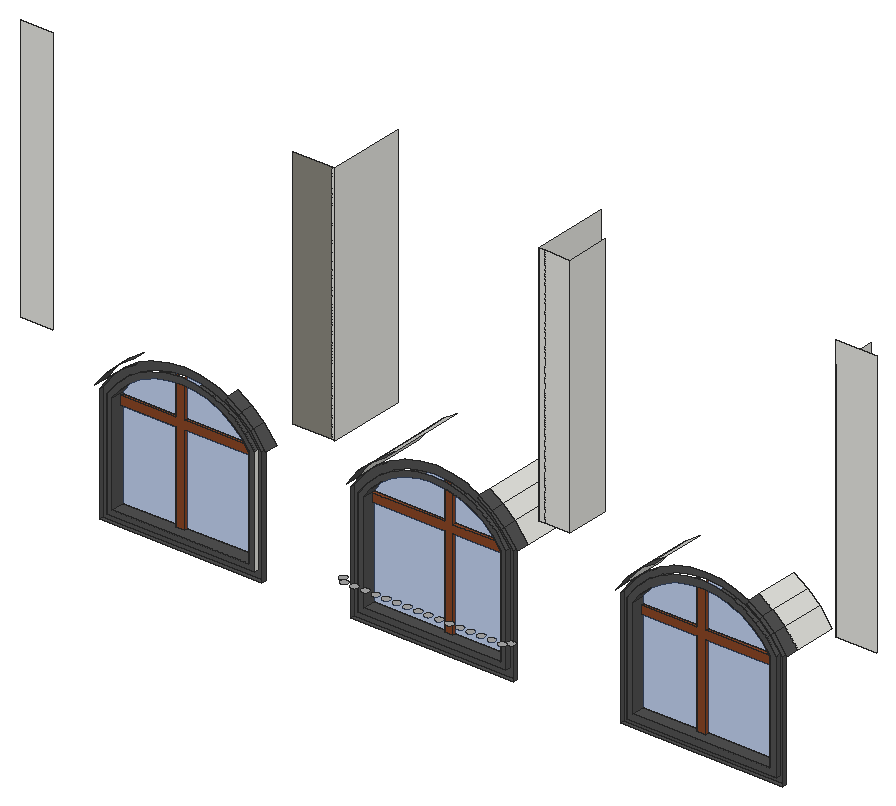
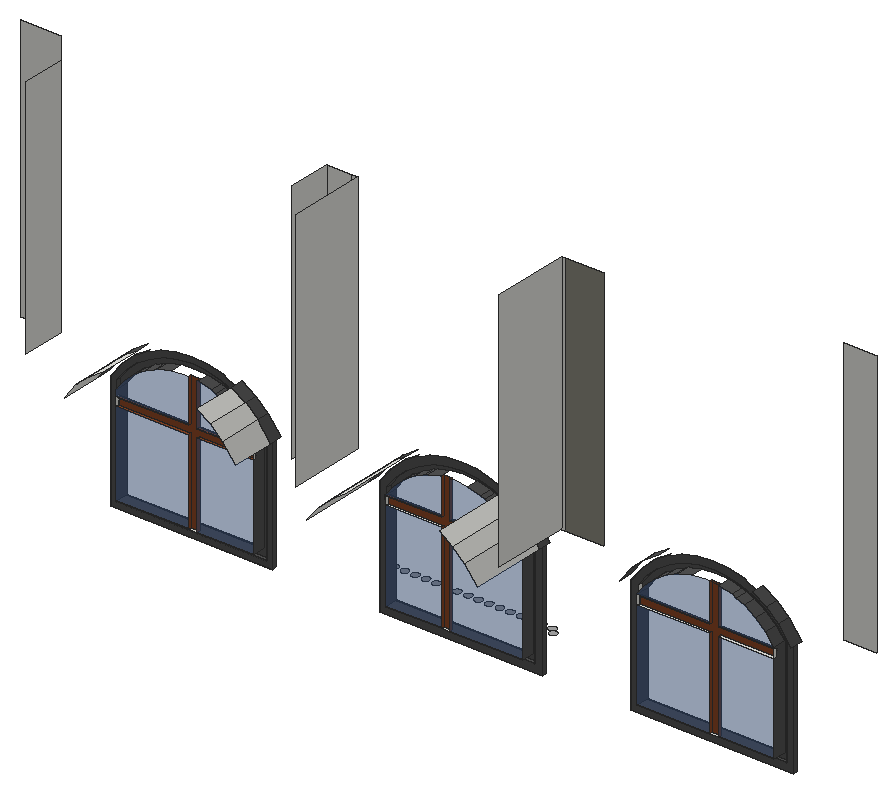
# SketchUp Ruby script. Lengths in inches.
U = 1.inch
M = Sketchup.active_model
def pt(a) = Geom::Point3d.new(a.map { |v| v * U })
def face(e, loops, mat)
  f = e.add_face(loops[0].map { |a| pt(a) })
  loops[1..].each { |l| e.add_face(l.map { |a| pt(a) }).erase! }
  f.material = f.back_material = mat if mat
  f
end
# faces: each face lists its corners as indices into pts; further lists are holes
def faces(e, pts, list, mat = nil) = list.each { |f| face(e, (f[0].is_a?(Array) ? f : [f]).map { |l| l.map { |i| pts[i] } }, mat) }
# xy, xz, yz: faces in a plane at the given z, y or x. An outline is a flat list of corners, or four numbers for a rectangle; further outlines are holes
def ring(l) = l.size == 4 ? [[l[0], l[1]], [l[2], l[1]], [l[2], l[3]], [l[0], l[3]]] : l.each_slice(2).to_a
def flat(e, list, mat, &to3) = list.each { |f| face(e, (f[0].is_a?(Array) ? f : [f]).map { |l| ring(l).map { |u, v| to3.(u, v) } }, mat) }
def xy(e, z, list, mat = nil) = flat(e, list, mat) { |x, y| [x, y, z] }
def xz(e, y, list, mat = nil) = flat(e, list, mat) { |x, z| [x, y, z] }
def yz(e, x, list, mat = nil) = flat(e, list, mat) { |y, z| [x, y, z] }
def lines(e, pts, list) = list.each { |a, b| e.add_line(pt(pts[a]), pt(pts[b])) }
# prism: a flat outline (further loops are holes) pulled along v
def prism(e, loops, v, mat = nil)
  f = face(e, loops, mat); d = Geom::Vector3d.new(v.map { |x| x * U })
  f.pushpull(f.normal.samedirection?(d) ? d.length : -d.length)
end
def box(e, o, s, mat = nil) = prism(e, [[o, [o[0] + s[0], o[1], o[2]], [o[0] + s[0], o[1] + s[1], o[2]], [o[0], o[1] + s[1], o[2]]]], [0, 0, s[2]], mat)
def at(x, y, z, deg = 0) = Geom::Transformation.translation(pt([x, y, z])) * Geom::Transformation.rotation(ORIGIN, Z_AXIS, deg.degrees)
def axes(o, x, y, z) = Geom::Transformation.new([*x, 0, *y, 0, *z, 0, *pt(o).to_a, 1])
def part(name) = M.definitions.add(name)
# library, detail: a bought-in or finely detailed component or shape, given as its bounding box
def library(name, o, s) = part(name).tap { |d| box(d.entities, o, s) }
def detail(e, o, s) = box(e.add_group.entities, o, s)
def put(e, d, t, mat = nil) = e.add_instance(d, t).tap { |i| i.material = mat if mat }
def group(e, t, mat = nil) = e.add_group.tap { |g| g.transformation = t; g.material = mat if mat }.entities
root = M.entities
M.materials.add("[0042_Sienna]").color = [137, 70, 38]
M.materials.add("[0132_LightGray]").color = [169, 169, 169]
M.materials.add("[0135_DarkGray]").color = [81, 81, 81]
M.materials.add("[Formica Graystone]").color = [137, 134, 124]
M.materials.add("[Translucent Glass Blue]").color = [66, 99, 158]
M.materials["[Translucent Glass Blue]"].alpha = 0.5
xy(root,498.46,[[244.93,40.6875,360.02,43.6875]],"[0135_DarkGray]")
xy(root,498.68,[[67.9,40.6875,182.55,43.6875]],"[0135_DarkGray]")
xy(root,498.79,[[435.27,40.6875,549.69,43.6875]],"[0135_DarkGray]")
xy(root,502.97,[[439.45,40.6875,545.51,43.6875]],"[0135_DarkGray]")
xy(root,503.78,[[73,40.6875,177.45,43.6875]],"[0135_DarkGray]")
xy(root,503.875,[[250.35,40.6875,354.6,43.6875]],"[0135_DarkGray]")
xy(root,507.66,[[116.29,47.6875,122.29,49.6875],[305.64,47.6875,311.64,49.6875],[483.7,47.6875,489.7,49.6875]])
xy(root,507.66,[[76.89,40.6875,173.57,40.6875,173.57,49.6875,122.29,49.6875,122.29,47.6875,116.29,47.6875,116.29,49.6875,76.89,49.6875],[254.14,40.6875,350.82,40.6875,350.82,49.6875,311.64,49.6875,311.64,47.6875,305.64,47.6875,305.64,49.6875,254.14,49.6875],[444.14,40.6875,540.82,40.6875,540.82,49.6875,489.7,49.6875,489.7,47.6875,483.7,47.6875,483.7,49.6875,444.14,49.6875]],"[0135_DarkGray]")
xy(root,523.91,[[245.54,31.88,246.17,31.96,246.76,32.21,247.26,32.6,247.65,33.1,247.89,33.6875,247.98,34.32,247.89,34.95,247.65,35.54,247.26,36.04,246.76,36.43,246.17,36.67,245.54,36.76,244.91,36.67,244.32,36.43,243.82,36.04,243.43,35.54,243.18,34.95,243.1,34.32,243.18,33.6875,243.43,33.1,243.82,32.6,244.32,32.21,244.91,31.96],[252.98,31.88,253.61,31.96,254.2,32.21,254.7,32.6,255.09,33.1,255.33,33.6875,255.41,34.32,255.33,34.95,255.09,35.54,254.7,36.04,254.2,36.43,253.61,36.67,252.98,36.76,252.35,36.67,251.76,36.43,251.25,36.04,250.87,35.54,250.62,34.95,250.54,34.32,250.62,33.6875,250.87,33.1,251.25,32.6,251.76,32.21,252.35,31.96],[260.41,31.88,261.04,31.96,261.63,32.21,262.14,32.6,262.53,33.1,262.77,33.6875,262.85,34.32,262.77,34.95,262.53,35.54,262.14,36.04,261.63,36.43,261.04,36.67,260.41,36.76,259.78,36.67,259.2,36.43,258.69,36.04,258.3,35.54,258.06,34.95,257.98,34.32,258.06,33.6875,258.3,33.1,258.69,32.6,259.2,32.21,259.78,31.96],[267.85,31.88,268.48,31.96,269.07,32.21,269.58,32.6,269.96,33.1,270.21,33.6875,270.29,34.32,270.21,34.95,269.96,35.54,269.58,36.04,269.07,36.43,268.48,36.67,267.85,36.76,267.22,36.67,266.63,36.43,266.13,36.04,265.74,35.54,265.5,34.95,265.41,34.32,265.5,33.6875,265.74,33.1,266.13,32.6,266.63,32.21,267.22,31.96],[275.29,31.88,275.92,31.96,276.51,32.21,277.01,32.6,277.4,33.1,277.64,33.6875,277.73,34.32,277.64,34.95,277.4,35.54,277.01,36.04,276.51,36.43,275.92,36.67,275.29,36.76,274.66,36.67,274.07,36.43,273.57,36.04,273.18,35.54,272.93,34.95,272.85,34.32,272.93,33.6875,273.18,33.1,273.57,32.6,274.07,32.21,274.66,31.96],
  [282.73,31.88,283.36,31.96,283.95,32.21,284.45,32.6,284.84,33.1,285.08,33.6875,285.16,34.32,285.08,34.95,284.84,35.54,284.45,36.04,283.95,36.43,283.36,36.67,282.73,36.76,282.1,36.67,281.51,36.43,281,36.04,280.62,35.54,280.37,34.95,280.29,34.32,280.37,33.6875,280.62,33.1,281,32.6,281.51,32.21,282.1,31.96],[290.16,31.88,290.79,31.96,291.38,32.21,291.89,32.6,292.28,33.1,292.52,33.6875,292.6,34.32,292.52,34.95,292.28,35.54,291.89,36.04,291.38,36.43,290.79,36.67,290.16,36.76,289.53,36.67,288.95,36.43,288.44,36.04,288.05,35.54,287.81,34.95,287.73,34.32,287.81,33.6875,288.05,33.1,288.44,32.6,288.95,32.21,289.53,31.96],[297.6,31.88,298.23,31.96,298.82,32.21,299.33,32.6,299.71,33.1,299.96,33.6875,300.04,34.32,299.96,34.95,299.71,35.54,299.33,36.04,298.82,36.43,298.23,36.67,297.6,36.76,296.97,36.67,296.38,36.43,295.88,36.04,295.49,35.54,295.25,34.95,295.16,34.32,295.25,33.6875,295.49,33.1,295.88,32.6,296.38,32.21,296.97,31.96],[305.04,31.88,305.67,31.96,306.26,32.21,306.76,32.6,307.15,33.1,307.39,33.6875,307.48,34.32,307.39,34.95,307.15,35.54,306.76,36.04,306.26,36.43,305.67,36.67,305.04,36.76,304.41,36.67,303.82,36.43,303.32,36.04,302.93,35.54,302.68,34.95,302.6,34.32,302.68,33.6875,302.93,33.1,303.32,32.6,303.82,32.21,304.41,31.96],[312.48,31.88,313.11,31.96,313.7,32.21,314.2,32.6,314.59,33.1,314.83,33.6875,314.91,34.32,314.83,34.95,314.59,35.54,314.2,36.04,313.7,36.43,313.11,36.67,312.48,36.76,311.85,36.67,311.26,36.43,310.75,36.04,310.37,35.54,310.12,34.95,310.04,34.32,310.12,33.6875,310.37,33.1,310.75,32.6,311.26,32.21,311.85,31.96],
  [319.91,31.88,320.54,31.96,321.13,32.21,321.64,32.6,322.03,33.1,322.27,33.6875,322.35,34.32,322.27,34.95,322.03,35.54,321.64,36.04,321.13,36.43,320.54,36.67,319.91,36.76,319.28,36.67,318.7,36.43,318.19,36.04,317.8,35.54,317.56,34.95,317.48,34.32,317.56,33.6875,317.8,33.1,318.19,32.6,318.7,32.21,319.28,31.96],[327.35,31.88,327.98,31.96,328.57,32.21,329.08,32.6,329.46,33.1,329.71,33.6875,329.79,34.32,329.71,34.95,329.46,35.54,329.08,36.04,328.57,36.43,327.98,36.67,327.35,36.76,326.72,36.67,326.13,36.43,325.63,36.04,325.24,35.54,325,34.95,324.91,34.32,325,33.6875,325.24,33.1,325.63,32.6,326.13,32.21,326.72,31.96],[334.79,31.88,335.42,31.96,336.01,32.21,336.51,32.6,336.9,33.1,337.14,33.6875,337.23,34.32,337.14,34.95,336.9,35.54,336.51,36.04,336.01,36.43,335.42,36.67,334.79,36.76,334.16,36.67,333.57,36.43,333.07,36.04,332.68,35.54,332.43,34.95,332.35,34.32,332.43,33.6875,332.68,33.1,333.07,32.6,333.57,32.21,334.16,31.96],[342.23,31.88,342.86,31.96,343.45,32.21,343.95,32.6,344.34,33.1,344.58,33.6875,344.66,34.32,344.58,34.95,344.34,35.54,343.95,36.04,343.45,36.43,342.86,36.67,342.23,36.76,341.6,36.67,341.01,36.43,340.5,36.04,340.12,35.54,339.87,34.95,339.79,34.32,339.87,33.6875,340.12,33.1,340.5,32.6,341.01,32.21,341.6,31.96],[349.66,31.88,350.29,31.96,350.88,32.21,351.39,32.6,351.78,33.1,352.02,33.6875,352.1,34.32,352.02,34.95,351.78,35.54,351.39,36.04,350.88,36.43,350.29,36.67,349.66,36.76,349.03,36.67,348.45,36.43,347.94,36.04,347.55,35.54,347.31,34.95,347.23,34.32,347.31,33.6875,347.55,33.1,347.94,32.6,348.45,32.21,349.03,31.96],
  [357.1,31.88,357.73,31.96,358.32,32.21,358.83,32.6,359.21,33.1,359.46,33.6875,359.54,34.32,359.46,34.95,359.21,35.54,358.83,36.04,358.32,36.43,357.73,36.67,357.1,36.76,356.47,36.67,355.88,36.43,355.38,36.04,354.99,35.54,354.75,34.95,354.66,34.32,354.75,33.6875,354.99,33.1,355.38,32.6,355.88,32.21,356.47,31.96],[241.96,35.55,242.59,35.64,243.18,35.88,243.6875,36.27,244.07,36.77,244.32,37.36,244.4,37.99,244.32,38.62,244.07,39.21,243.6875,39.71,243.18,40.1,242.59,40.34,241.96,40.43,241.33,40.34,240.74,40.1,240.24,39.71,239.85,39.21,239.61,38.62,239.52,37.99,239.61,37.36,239.85,36.77,240.24,36.27,240.74,35.88,241.33,35.64],[360.59,35.72,361.22,35.81,361.8,36.05,362.31,36.4375,362.7,36.94,362.94,37.53,363.02,38.16,362.94,38.79,362.7,39.38,362.31,39.89,361.8,40.27,361.22,40.52,360.59,40.6,359.96,40.52,359.37,40.27,358.86,39.89,358.48,39.38,358.23,38.79,358.15,38.16,358.23,37.53,358.48,36.94,358.86,36.4375,359.37,36.05,359.96,35.81]],"[0132_LightGray]")
xy(root,567.47,[[444.14,47.6875,483.7,49.6875],[489.7,47.6875,540.82,49.6875]],"[0042_Sienna]")
xy(root,570.97,[[76.89,47.6875,116.29,49.6875],[122.29,47.6875,173.57,49.6875]])
xy(root,571.72,[[254.14,47.6875,305.64,49.6875],[311.64,47.6875,350.82,49.6875]])
xy(root,573.47,[[444.14,47.6875,483.7,49.6875],[489.7,47.6875,540.82,49.6875]],"[0042_Sienna]")
xy(root,576.97,[[76.89,47.6875,116.29,49.6875],[122.29,47.6875,173.57,49.6875]],"[0042_Sienna]")
xy(root,577.72,[[254.14,47.6875,305.64,49.6875],[311.64,47.6875,350.82,49.6875]],"[0042_Sienna]")
xz(root,40.6875,[[[439.45,502.97,545.51,502.97,545.51,579.58,538.47,588.73,530.9,595.77,522.26,601.46,515.85,604.29,512.8,605.64,502.78,608.1875,492.48,609.05,482.17,608.1875,472.16,605.64,469.1,604.29,462.7,601.46,454.0625,595.77,446.49,588.73,439.45,579.58],[444.14,507.66,444.14,577.99,449.96,585.57,456.97,592.07,464.95,597.33,471,600,473.69,601.19,482.95,603.55,492.48,604.35,502,603.55,511.27,601.19,513.96,600,520.01,597.33,527.99,592.07,534.99,585.57,540.82,577.99,540.82,507.66]],[[73,503.78,177.45,503.78,177.45,579.3125,170.625,588.1875,163.15,595.14,154.625,600.75,148.28,603.55,145.29,604.87,135.4,607.39,125.23,608.24,115.06,607.39,105.17,604.87,102.18,603.55,95.83,600.75,87.31,595.14,79.83,588.1875,73,579.3125],[76.89,507.66,76.89,577.99,82.71,585.57,89.72,592.07,97.7,597.33,103.75,600,106.44,601.19,115.7,603.55,125.23,604.35,134.75,603.55,144.02,601.19,146.71,600,152.76,597.33,160.74,592.07,167.74,585.57,173.57,577.99,173.57,507.66]],[[250.35,503.875,354.6,503.875,354.6,579.28,347.8,588.12,340.34,595.06,331.83,600.66,325.49,603.46,322.51,604.78,312.63,607.29,302.48,608.14,292.33,607.29,282.45,604.78,279.47,603.46,273.13,600.66,264.62,595.06,257.16,588.12,250.35,579.28],[254.14,507.66,254.14,577.99,259.96,585.57,266.97,592.07,274.95,597.33,281,600,283.69,601.19,292.95,603.55,302.48,604.35,312,603.55,321.27,601.19,323.96,600,330.01,597.33,337.99,592.07,344.99,585.57,350.82,577.99,350.82,507.66]]],"[0135_DarkGray]")
xz(root,43.6875,[[[244.93,498.46,360.02,498.46,360.02,581.12,351.82,591.78,343.69,599.34,334.43,605.4375,327.68,608.42,324.28,609.92,313.53,612.66,302.48,613.58,291.42,612.66,280.68,609.92,277.28,608.42,270.53,605.4375,261.26,599.34,253.14,591.78,244.93,581.12],[250.35,503.875,250.35,579.28,257.16,588.12,264.62,595.06,273.13,600.66,279.47,603.46,282.45,604.78,292.33,607.29,302.48,608.14,312.63,607.29,322.51,604.78,325.49,603.46,331.83,600.66,340.34,595.06,347.8,588.12,354.6,579.28,354.6,503.875]],[[67.9,498.68,182.55,498.68,182.55,581.05,174.41,591.64,166.31,599.16,157.07,605.24,150.34,608.22,146.96,609.71,136.25,612.4375,125.23,613.36,114.21,612.4375,103.5,609.71,100.12,608.22,93.38,605.24,84.15,599.16,76.05,591.64,67.9,581.05],[73,503.78,73,579.3125,79.83,588.1875,87.31,595.14,95.83,600.75,102.18,603.55,105.17,604.87,115.06,607.39,125.23,608.24,135.4,607.39,145.29,604.87,148.28,603.55,154.625,600.75,163.15,595.14,170.625,588.1875,177.45,579.3125,177.45,503.78]],[[435.27,498.79,549.69,498.79,549.69,581.01,541.57,591.5625,533.49,599.07,524.27,605.14,517.54,608.11,514.17,609.6,503.48,612.33,492.48,613.25,481.48,612.33,470.78,609.6,467.41,608.11,460.6875,605.14,451.47,599.07,443.38,591.5625,435.27,581.01],[439.45,502.97,439.45,579.58,446.49,588.73,454.0625,595.77,462.7,601.46,469.1,604.29,472.16,605.64,482.17,608.1875,492.48,609.05,502.78,608.1875,512.8,605.64,515.85,604.29,522.26,601.46,530.9,595.77,538.47,588.73,545.51,579.58,545.51,502.97]]],"[0135_DarkGray]")
xz(root,47.6875,[[116.29,507.66,122.29,507.66,122.29,570.97,173.57,570.97,173.57,576.97,122.29,576.97,122.29,604.1,116.29,603.55,116.29,576.97,76.89,576.97,76.89,570.97,116.29,570.97],[305.64,507.66,311.64,507.66,311.64,571.72,350.82,571.72,350.82,577.72,311.64,577.72,311.64,603.58,305.64,604.08,305.64,577.72,254.14,577.72,254.14,571.72,305.64,571.72],[483.7,507.66,489.7,507.66,489.7,567.47,540.82,567.47,540.82,573.47,489.7,573.47,489.7,604.11,483.7,603.61,483.7,573.47,444.14,573.47,444.14,567.47,483.7,567.47]],"[0042_Sienna]")
xz(root,49.6875,[[350.82,571.72,350.82,577.72,351.51,577.72],[4.9375,600,27.68,787.6875],[224.47,600,226.6,772.09],[226.6,600,227.04,772.09],[370.55,600,370.74,772.09],
  [370.74,600,374.55,772.09],[374.55,600,392.7,772.09],[580.01,600,608.5,787.6875]])
xz(root,49.6875,[[197.35,600,224.47,772.09]],"[Formica Graystone]")
xz(root,49.6875,[[76.89,507.66,116.29,570.97],[122.29,507.66,173.57,570.97],[254.14,507.66,305.64,571.72],[311.64,507.66,350.82,571.72],[444.14,507.66,483.7,567.47],
  [489.7,507.66,540.82,567.47],[444.14,573.47,483.7,573.47,483.7,603.61,482.95,603.55,473.69,601.19,471,600,464.95,597.33,456.97,592.07,449.96,585.57,444.14,577.99],[489.7,573.47,540.82,573.47,540.82,577.99,534.99,585.57,527.99,592.07,520.01,597.33,513.96,600,511.27,601.19,502,603.55,492.48,604.35,489.7,604.11],[76.89,576.97,116.29,576.97,116.29,603.55,122.29,604.1,115.7,603.55,106.44,601.19,103.75,600,97.7,597.33,89.72,592.07,82.71,585.57,76.89,577.99],[122.29,576.97,173.57,576.97,173.57,577.99,167.74,585.57,160.74,592.07,152.76,597.33,146.71,600,144.02,601.19,134.75,603.55,125.23,604.35,122.29,604.1],
  [254.14,577.72,305.64,577.72,305.64,604.08,302.48,604.35,292.95,603.55,283.69,601.19,281,600,274.95,597.33,266.97,592.07,259.96,585.57,254.14,577.99],[311.64,577.72,350.82,577.72,350.82,577.99,344.99,585.57,337.99,592.07,330.01,597.33,323.96,600,321.27,601.19,312,603.55,311.64,603.58]],"[Translucent Glass Blue]")
yz(root,67.9,[[40.6875,498.68,43.6875,581.05]],"[0135_DarkGray]")
yz(root,73,[[40.6875,503.78,43.6875,579.3125]],"[0135_DarkGray]")
yz(root,76.89,[[47.6875,570.97,49.6875,576.97]])
yz(root,76.89,[[40.6875,507.66,49.6875,507.66,49.6875,570.97,47.6875,570.97,47.6875,576.97,49.6875,576.97,49.6875,577.99,40.6875,577.99]],"[0135_DarkGray]")
yz(root,116.29,[[47.6875,507.66,49.6875,570.97],[47.6875,576.97,49.6875,603.55]],"[0042_Sienna]")
yz(root,122.29,[[47.6875,507.66,49.6875,570.97],[47.6875,576.97,49.6875,604.1]],"[0042_Sienna]")
yz(root,173.57,[[47.6875,570.97,49.6875,576.97]])
yz(root,173.57,[[40.6875,507.66,40.6875,577.99,49.6875,577.99,49.6875,576.97,47.6875,576.97,47.6875,570.97,49.6875,570.97,49.6875,507.66]],"[0135_DarkGray]")
yz(root,177.45,[[40.6875,503.78,43.6875,579.3125]])
yz(root,182.55,[[40.6875,498.68,43.6875,581.05]],"[0135_DarkGray]")
yz(root,227.04,[[49.6875,600,104.375,772.09]])
yz(root,244.93,[[40.6875,498.46,43.6875,581.12]],"[0135_DarkGray]")
yz(root,250.35,[[40.6875,503.875,43.6875,579.28]],"[0135_DarkGray]")
yz(root,254.14,[[47.6875,571.72,49.6875,577.72]])
yz(root,254.14,[[40.6875,507.66,49.6875,507.66,49.6875,571.72,47.6875,571.72,47.6875,577.72,49.6875,577.72,49.6875,577.99,40.6875,577.99]],"[0135_DarkGray]")
yz(root,305.64,[[47.6875,507.66,49.6875,571.72],[47.6875,577.72,49.6875,604.08]],"[0042_Sienna]")
yz(root,311.64,[[47.6875,507.66,49.6875,571.72],[47.6875,577.72,49.6875,603.58]],"[0042_Sienna]")
yz(root,350.82,[[47.6875,571.72,49.6875,577.72]])
yz(root,350.82,[[40.6875,507.66,40.6875,577.99,49.6875,577.99,49.6875,577.72,47.6875,577.72,47.6875,571.72,49.6875,571.72,49.6875,507.66]],"[0135_DarkGray]")
yz(root,354.6,[[40.6875,503.875,43.6875,579.28]],"[0135_DarkGray]")
yz(root,360.02,[[40.6875,498.46,43.6875,581.12]],"[0135_DarkGray]")
yz(root,370.55,[[49.6875,600,104.375,772.09]])
yz(root,392.7,[[49.6875,600,80.4375,772.09]])
yz(root,435.27,[[40.6875,498.79,43.6875,581.01]],"[0135_DarkGray]")
yz(root,439.45,[[40.6875,502.97,43.6875,579.58]],"[0135_DarkGray]")
yz(root,444.14,[[47.6875,567.47,49.6875,573.47]])
yz(root,444.14,[[40.6875,507.66,49.6875,507.66,49.6875,567.47,47.6875,567.47,47.6875,573.47,49.6875,573.47,49.6875,577.99,40.6875,577.99]],"[0135_DarkGray]")
yz(root,483.7,[[47.6875,507.66,49.6875,567.47],[47.6875,573.47,49.6875,603.61]],"[0042_Sienna]")
yz(root,489.7,[[47.6875,507.66,49.6875,567.47],[47.6875,573.47,49.6875,604.11]],"[0042_Sienna]")
yz(root,540.82,[[47.6875,567.47,49.6875,573.47]])
yz(root,540.82,[[40.6875,507.66,40.6875,577.99,49.6875,577.99,49.6875,573.47,47.6875,573.47,47.6875,567.47,49.6875,567.47,49.6875,507.66]],"[0135_DarkGray]")
yz(root,545.51,[[40.6875,502.97,43.6875,579.58]],"[0135_DarkGray]")
yz(root,549.69,[[40.6875,498.79,43.6875,581.01]],"[0135_DarkGray]")
yz(root,580.01,[[49.6875,600,80.4375,772.09]])
p = [[76.89,49.6875,577.99],[82.71,49.6875,585.57],[82.71,40.6875,585.57],[76.89,40.6875,577.99],[167.74,49.6875,585.57],[173.57,49.6875,577.99],
  [173.57,40.6875,577.99],[167.74,40.6875,585.57],[254.14,49.6875,577.99],[259.96,49.6875,585.57],[259.96,40.6875,585.57],[254.14,40.6875,577.99],
  [344.99,49.6875,585.57],[350.82,49.6875,577.99],[350.82,40.6875,577.99],[344.99,40.6875,585.57],[444.14,49.6875,577.99],[449.96,49.6875,585.57],
  [449.96,40.6875,585.57],[444.14,40.6875,577.99],[534.99,49.6875,585.57],[540.82,49.6875,577.99],[540.82,40.6875,577.99],[534.99,40.6875,585.57],
  [79.83,43.6875,588.1875],[73,43.6875,579.3125],[73,40.6875,579.3125],[79.83,40.6875,588.1875],[177.45,43.6875,579.3125],[170.625,43.6875,588.1875],
  [170.625,40.6875,588.1875],[177.45,40.6875,579.3125],[257.16,43.6875,588.12],[250.35,43.6875,579.28],[250.35,40.6875,579.28],[257.16,40.6875,588.12],
  [354.6,43.6875,579.28],[347.8,43.6875,588.12],[347.8,40.6875,588.12],[354.6,40.6875,579.28],[446.49,43.6875,588.73],[439.45,43.6875,579.58],
  [439.45,40.6875,579.58],[446.49,40.6875,588.73],[545.51,43.6875,579.58],[538.47,43.6875,588.73],[538.47,40.6875,588.73],[545.51,40.6875,579.58],
  [67.9,43.6875,581.05],[76.05,43.6875,591.64],[76.05,40.6875,591.64],[67.9,40.6875,581.05],[174.41,43.6875,591.64],[182.55,43.6875,581.05],
  [182.55,40.6875,581.05],[174.41,40.6875,591.64],[435.27,43.6875,581.01],[443.38,43.6875,591.5625],[443.38,40.6875,591.5625],[435.27,40.6875,581.01],
  [541.57,43.6875,591.5625],[549.69,43.6875,581.01],[549.69,40.6875,581.01],[541.57,40.6875,591.5625],[244.93,43.6875,581.12],[253.14,43.6875,591.78],
  [253.14,40.6875,591.78],[244.93,40.6875,581.12],[351.82,43.6875,591.78],[360.02,43.6875,581.12],[360.02,40.6875,581.12],[351.82,40.6875,591.78],
  [73.8125,49.6875,593.68],[64.89,49.6875,582.07],[64.89,40.6875,582.07],[73.8125,40.6875,593.68],[185.57,49.6875,582.07],[176.65,49.6875,593.68],
  [176.65,40.6875,593.68],[185.57,40.6875,582.07],[251.0625,49.6875,593.68],[242.14,49.6875,582.07],[242.14,40.6875,582.07],[251.0625,40.6875,593.68],
  [362.82,49.6875,582.07],[353.9,49.6875,593.68],[353.9,40.6875,593.68],[362.82,40.6875,582.07],[432.14,49.6875,582.07],[441.0625,49.6875,593.68],
  [441.0625,40.6875,593.68],[432.14,40.6875,582.07],[543.9,49.6875,593.68],[552.82,49.6875,582.07],[552.82,40.6875,582.07],[543.9,40.6875,593.68],
  [242.14,104.375,582.07],[251.0625,104.375,593.68],[353.9,104.375,593.68],[362.82,104.375,582.07],[432.14,80.4375,582.07],[441.0625,80.4375,593.68],
  [543.9,80.4375,593.68],[552.82,80.4375,582.07],[89.72,49.6875,592.07],[89.72,40.6875,592.07],[160.74,49.6875,592.07],[160.74,40.6875,592.07],
  [266.97,49.6875,592.07],[266.97,40.6875,592.07],[337.99,49.6875,592.07],[337.99,40.6875,592.07],[456.97,49.6875,592.07],[456.97,40.6875,592.07],
  [527.99,49.6875,592.07],[527.99,40.6875,592.07],[264.62,43.6875,595.06],[264.62,40.6875,595.06],[340.34,43.6875,595.06],[340.34,40.6875,595.06],
  [87.31,43.6875,595.14],[87.31,40.6875,595.14],[163.15,43.6875,595.14],[163.15,40.6875,595.14],[454.0625,43.6875,595.77],[454.0625,40.6875,595.77],
  [530.9,43.6875,595.77],[530.9,40.6875,595.77],[84.15,43.6875,599.16],[84.15,40.6875,599.16],[166.31,43.6875,599.16],[166.31,40.6875,599.16],
  [451.47,43.6875,599.07],[451.47,40.6875,599.07],[533.49,43.6875,599.07],[533.49,40.6875,599.07],[261.26,43.6875,599.34],[261.26,40.6875,599.34],
  [343.69,43.6875,599.34],[343.69,40.6875,599.34],[97.7,49.6875,597.33],[97.7,40.6875,597.33],[152.76,49.6875,597.33],[152.76,40.6875,597.33],
  [274.95,49.6875,597.33],[274.95,40.6875,597.33],[330.01,49.6875,597.33],[330.01,40.6875,597.33],[464.95,49.6875,597.33],[464.95,40.6875,597.33],
  [520.01,49.6875,597.33],[520.01,40.6875,597.33],[82.28,49.6875,601.54],[82.28,40.6875,601.54],[168.18,49.6875,601.54],[168.18,40.6875,601.54],
  [259.53,49.6875,601.54],[259.53,40.6875,601.54],[345.43,49.6875,601.54],[345.43,40.6875,601.54],[449.53,49.6875,601.54],[449.53,40.6875,601.54],
  [535.43,49.6875,601.54],[535.43,40.6875,601.54],[259.53,104.375,601.54],[345.43,104.375,601.54],[449.53,80.4375,601.54],[535.43,80.4375,601.54],
  [95.83,43.6875,600.75],[95.83,40.6875,600.75],[154.625,43.6875,600.75],[154.625,40.6875,600.75],[273.13,43.6875,600.66],[273.13,40.6875,600.66],
  [331.83,43.6875,600.66],[331.83,40.6875,600.66],[462.7,43.6875,601.46],[462.7,40.6875,601.46],[522.26,43.6875,601.46],[522.26,40.6875,601.46],
  [103.75,49.6875,600],[103.75,40.6875,600],[146.71,49.6875,600],[146.71,40.6875,600],[281,49.6875,600],[281,40.6875,600],
  [323.96,49.6875,600],[323.96,40.6875,600],[471,49.6875,600],[471,40.6875,600],[513.96,49.6875,600],[513.96,40.6875,600],
  [460.6875,43.6875,605.14],[460.6875,40.6875,605.14],[524.27,43.6875,605.14],[524.27,40.6875,605.14],[93.38,43.6875,605.24],[93.38,40.6875,605.24],
  [157.07,43.6875,605.24],[157.07,40.6875,605.24],[270.53,43.6875,605.4375],[270.53,40.6875,605.4375],[334.43,43.6875,605.4375],[334.43,40.6875,605.4375],
  [106.44,49.6875,601.19],[106.44,40.6875,601.19],[144.02,49.6875,601.19],[144.02,40.6875,601.19],[283.69,49.6875,601.19],[283.69,40.6875,601.19],
  [321.27,49.6875,601.19],[321.27,40.6875,601.19],[473.69,49.6875,601.19],[473.69,40.6875,601.19],[511.27,49.6875,601.19],[511.27,40.6875,601.19],
  [102.18,43.6875,603.55],[102.18,40.6875,603.55],[148.28,43.6875,603.55],[148.28,40.6875,603.55],[279.47,43.6875,603.46],[279.47,40.6875,603.46],
  [325.49,43.6875,603.46],[325.49,40.6875,603.46],[115.7,49.6875,603.55],[115.7,40.6875,603.55],[134.75,49.6875,603.55],[134.75,40.6875,603.55],
  [292.95,49.6875,603.55],[292.95,40.6875,603.55],[312,49.6875,603.55],[312,40.6875,603.55],[482.95,49.6875,603.55],[482.95,40.6875,603.55],
  [502,49.6875,603.55],[502,40.6875,603.55],[91.93,49.6875,607.9],[91.93,40.6875,607.9],[158.52,49.6875,607.9],[158.52,40.6875,607.9],
  [269.18,49.6875,607.9],[269.18,40.6875,607.9],[335.77,49.6875,607.9],[335.77,40.6875,607.9],[459.18,49.6875,607.9],[459.18,40.6875,607.9],
  [469.1,43.6875,604.29],[469.1,40.6875,604.29],[515.85,43.6875,604.29],[515.85,40.6875,604.29],[525.77,49.6875,607.9],[525.77,40.6875,607.9],
  [269.18,104.375,607.9],[335.77,104.375,607.9],[459.18,80.4375,607.9],[525.77,80.4375,607.9]]
faces(root,p,[[0,1,2,3],[4,5,6,7],[8,9,10,11],[12,13,14,15],[16,17,18,19],[20,21,22,23],[24,25,26,27],[28,29,30,31],
  [32,33,34,35],[36,37,38,39],[40,41,42,43],[44,45,46,47],[48,49,50,51],[52,53,54,55],[56,57,58,59],[60,61,62,63],
  [64,65,66,67],[68,69,70,71],[72,73,74,75],[76,77,78,79],[80,81,82,83],[84,85,86,87],[88,89,90,91],[92,93,94,95],
  [1,104,105,2],[106,4,7,107],[9,108,109,10],[110,12,15,111],[17,112,113,18],[114,20,23,115],[116,32,35,117],[37,118,119,38],
  [120,24,27,121],[29,122,123,30],[124,40,43,125],[45,126,127,46],[49,128,129,50],[130,52,55,131],[57,132,133,58],[134,60,63,135],
  [65,136,137,66],[138,68,71,139],[104,140,141,105],[142,106,107,143],[108,144,145,109],[146,110,111,147],[112,148,149,113],[150,114,115,151],
  [152,72,75,153],[77,154,155,78],[156,80,83,157],[85,158,159,86],[89,160,161,90],[162,92,95,163],[168,120,121,169],[122,170,171,123],
  [172,116,117,173],[118,174,175,119],[176,124,125,177],[126,178,179,127],[140,180,181,141],[182,142,143,183],[144,184,185,145],[186,146,147,187],
  [148,188,189,149],[190,150,151,191],[132,192,193,133],[194,134,135,195],[128,196,197,129],[198,130,131,199],[136,200,201,137],[202,138,139,203],
  [180,204,205,181],[206,182,183,207],[184,208,209,185],[210,186,187,211],[188,212,213,189],[214,190,191,215],[216,168,169,217],[170,218,219,171],
  [220,172,173,221],[174,222,223,175],[204,224,225,205],[226,206,207,227],[208,228,229,209],[230,210,211,231],[212,232,233,213],[234,214,215,235],
  [236,152,153,237],[154,238,239,155],[240,156,157,241],[158,242,243,159],[160,244,245,161],[246,176,177,247],[178,248,249,179],[250,162,163,251]],"[0135_DarkGray]")
faces(root,p,[[80,81,96,97],[84,85,98,99],[89,88,100,101],[93,92,102,103],[156,80,97,164],[85,158,165,98],[160,89,101,166],[92,162,167,102],
  [240,156,164,252],[158,242,253,165],[244,160,166,254],[162,250,255,167]])
